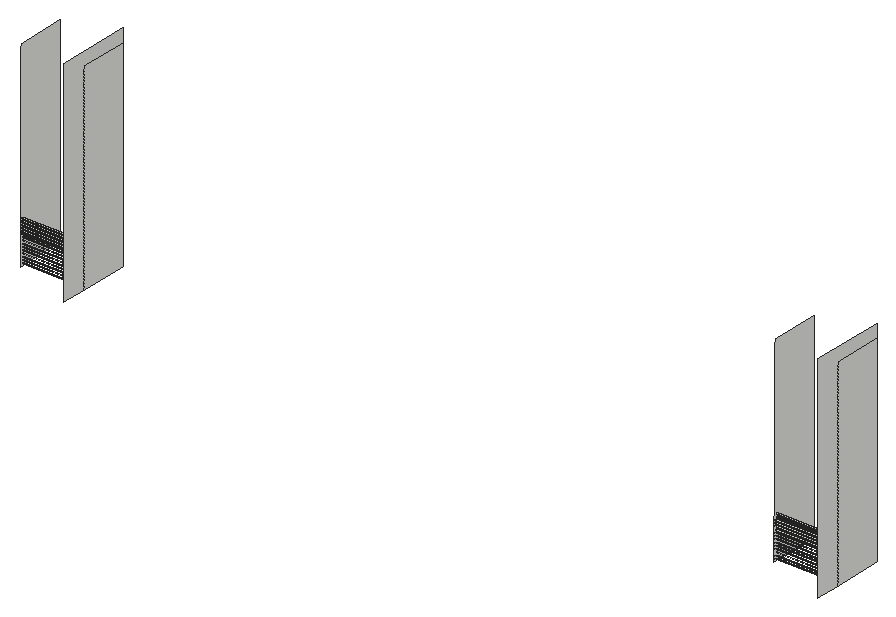
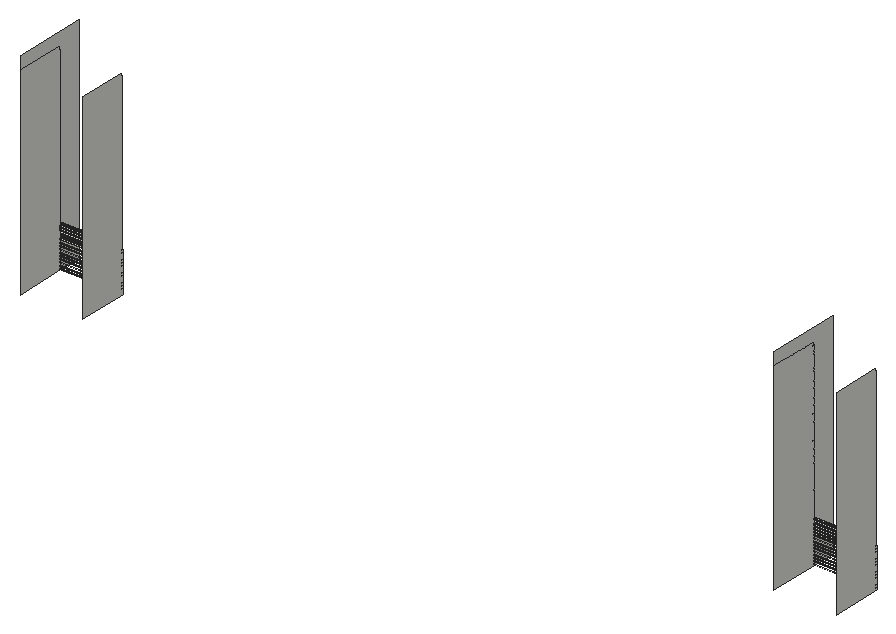
# SketchUp Ruby script. Lengths in inches.
U = 1.inch
M = Sketchup.active_model
def pt(a) = Geom::Point3d.new(a.map { |v| v * U })
def face(e, loops, mat)
  f = e.add_face(loops[0].map { |a| pt(a) })
  loops[1..].each { |l| e.add_face(l.map { |a| pt(a) }).erase! }
  f.material = f.back_material = mat if mat
  f
end
# faces: each face lists its corners as indices into pts; further lists are holes
def faces(e, pts, list, mat = nil) = list.each { |f| face(e, (f[0].is_a?(Array) ? f : [f]).map { |l| l.map { |i| pts[i] } }, mat) }
# xy, xz, yz: faces in a plane at the given z, y or x. An outline is a flat list of corners, or four numbers for a rectangle; further outlines are holes
def ring(l) = l.size == 4 ? [[l[0], l[1]], [l[2], l[1]], [l[2], l[3]], [l[0], l[3]]] : l.each_slice(2).to_a
def flat(e, list, mat, &to3) = list.each { |f| face(e, (f[0].is_a?(Array) ? f : [f]).map { |l| ring(l).map { |u, v| to3.(u, v) } }, mat) }
def xy(e, z, list, mat = nil) = flat(e, list, mat) { |x, y| [x, y, z] }
def xz(e, y, list, mat = nil) = flat(e, list, mat) { |x, z| [x, y, z] }
def yz(e, x, list, mat = nil) = flat(e, list, mat) { |y, z| [x, y, z] }
def lines(e, pts, list) = list.each { |a, b| e.add_line(pt(pts[a]), pt(pts[b])) }
# prism: a flat outline (further loops are holes) pulled along v
def prism(e, loops, v, mat = nil)
  f = face(e, loops, mat); d = Geom::Vector3d.new(v.map { |x| x * U })
  f.pushpull(f.normal.samedirection?(d) ? d.length : -d.length)
end
def box(e, o, s, mat = nil) = prism(e, [[o, [o[0] + s[0], o[1], o[2]], [o[0] + s[0], o[1] + s[1], o[2]], [o[0], o[1] + s[1], o[2]]]], [0, 0, s[2]], mat)
def at(x, y, z, deg = 0) = Geom::Transformation.translation(pt([x, y, z])) * Geom::Transformation.rotation(ORIGIN, Z_AXIS, deg.degrees)
def axes(o, x, y, z) = Geom::Transformation.new([*x, 0, *y, 0, *z, 0, *pt(o).to_a, 1])
def part(name) = M.definitions.add(name)
# library, detail: a bought-in or finely detailed component or shape, given as its bounding box
def library(name, o, s) = part(name).tap { |d| box(d.entities, o, s) }
def detail(e, o, s) = box(e.add_group.entities, o, s)
def put(e, d, t, mat = nil) = e.add_instance(d, t).tap { |i| i.material = mat if mat }
def group(e, t, mat = nil) = e.add_group.tap { |g| g.transformation = t; g.material = mat if mat }.entities
root = M.entities
xy(root,243.875,[[533.89,1125.04,620.51,1127.73],[1582.21,1125.04,1668.82,1127.73]])
xy(root,246.91,[[533.89,1125.04,620.51,1127.73],[1582.21,1125.04,1668.82,1127.73]])
xy(root,247.9375,[[533.89,1125.04,620.51,1127.73],[1582.21,1125.04,1668.82,1127.73]])
xy(root,250.97,[[533.89,1125.04,620.51,1127.73],[1582.21,1125.04,1668.82,1127.73]])
xy(root,252,[[533.89,1125.04,620.51,1127.73],[1582.21,1125.04,1668.82,1127.73]])
xy(root,255.03,[[533.89,1125.04,620.51,1127.73],[1582.21,1125.04,1668.82,1127.73]])
xy(root,256.0625,[[533.89,1125.04,620.51,1127.73],[1582.21,1125.04,1668.82,1127.73]])
xy(root,259.09,[[533.89,1125.04,620.51,1127.73],[1582.21,1125.04,1668.82,1127.73]])
xy(root,260.125,[[533.89,1125.42,620.51,1127.73],[1582.21,1125.42,1668.82,1127.73]])
xy(root,263.16,[[533.89,1125.42,620.51,1127.73],[1582.21,1125.42,1668.82,1127.73]])
xy(root,264.1875,[[533.89,1125.42,620.51,1127.73],[1582.21,1125.42,1668.82,1127.73]])
xz(root,1127.73,[[533.89,206.47,620.51,207.375],[1582.21,206.47,1668.82,207.375],[533.89,210.41,620.51,211.375],[1582.21,210.41,1668.82,211.375],[533.89,214.41,620.51,215.4375],
  [1582.21,214.41,1668.82,215.4375],[533.89,218.47,620.51,219.5],[1582.21,218.47,1668.82,219.5],[533.89,222.53,620.51,223.5625],[1582.21,222.53,1668.82,223.5625],
  [533.89,226.59,620.51,227.625],[1582.21,226.59,1668.82,227.625],[533.89,230.66,620.51,231.6875],[1582.21,230.66,1668.82,231.6875],[533.89,234.72,620.51,235.75],
  [1582.21,234.72,1668.82,235.75],[533.89,238.78,620.51,239.8125],[1582.21,238.78,1668.82,239.8125],[533.89,242.84,620.51,243.875]])
yz(root,533.89,[[1125.04,203.4375,1125.04,206.47,1127.73,206.47,1127.73,207.375,1125.04,207.375,1125.04,210.41,1127.73,210.41,1127.73,211.375,1125.04,211.375,1125.04,214.41,1127.73,214.41,1127.73,215.4375,1125.04,215.4375,1125.04,218.47,1127.73,218.47,1127.73,219.5,1125.04,219.5,1125.04,222.53,1127.73,222.53,1127.73,223.5625,1125.04,223.5625,1125.04,226.59,1127.73,226.59,1127.73,227.625,1125.04,227.625,1125.04,230.66,1127.73,230.66,1127.73,231.6875,1125.04,231.6875,1125.04,234.72,1127.73,234.72,1127.73,235.75,1125.04,235.75,1125.04,238.78,1127.73,238.78,1127.73,239.8125,1125.04,239.8125,1125.04,242.84,1127.73,242.84,1127.73,243.875,1125.04,243.875,1125.04,246.91,1127.73,246.91,1127.73,247.9375,1125.04,247.9375,1125.04,250.97,1127.73,250.97,1127.73,252,1125.04,252,1125.04,255.03,1127.73,255.03,1127.73,256.0625,1125.04,256.0625,1125.04,259.09,1127.73,259.09,1127.73,260.125,1125.42,260.125,1125.42,263.16,1127.73,263.16,1127.73,264.1875,1125.42,264.1875,1125.42,267.22,1127.73,267.22,1127.73,268.25,1125.42,268.25,1125.42,271.28,1127.73,271.28,1127.73,272.3125,1125.42,272.3125,1125.42,275.34,1127.73,275.34,1127.73,276.375,1125.42,276.375,1125.42,279.41,1127.73,279.41,1127.73,280.4375,1125.42,280.4375,1125.42,283.47,1127.73,283.47,1127.73,284.5,1125.42,284.5,1125.42,287.53,1127.73,287.53,1127.73,288.5625,1125.42,288.5625,1125.42,291.59,1127.73,291.59,1127.73,292.625,1125.42,292.625,1125.42,295.66,1127.73,295.66,1127.73,296.6875,1125.42,296.6875,1125.42,299.72,1127.73,299.72,1127.73,300.75,1125.42,300.75,1125.42,303.78,1127.73,303.78,1127.73,304.8125,1125.42,304.8125,1125.42,307.84,1127.73,307.84,1127.73,308.875,1125.42,308.875,1125.42,311.91,1127.73,311.91,1127.73,312.9375,1125.42,312.9375,1125.42,315.97,1127.73,315.97,1127.73,317,1125.42,317,1125.42,320.03,1127.73,320.03,1127.73,321.0625,1125.42,321.0625,1125.42,324.09,1127.73,324.09,1127.73,325.125,1125.42,325.125,1125.42,328.16,1127.73,328.16,1127.73,329.1875,1125.42,329.1875,1125.42,332.22,1127.73,332.22,1127.73,333.25,1125.42,333.25,1125.42,336.28,1127.73,336.28,1127.73,337.3125,1125.42,337.3125,1125.42,340.34,1127.73,340.34,1127.73,341.375,1125.42,341.375,1125.42,344.41,1127.73,344.41,1127.73,345.4375,1125.42,345.4375,1125.42,348.47,1127.73,348.47,1127.73,349.5,1125.42,349.5,1125.42,352.53,1127.73,352.53,1127.73,353.5625,1125.42,353.5625,1125.42,356.59,1127.73,356.59,1127.73,357.625,1125.42,357.625,1125.42,360.66,1127.73,360.66,1127.73,361.6875,1125.42,361.6875,1125.42,364.72,1127.73,364.72,1127.73,365.75,1125.42,365.75,1125.42,368.78,1127.73,368.78,1127.73,369.8125,1125.42,369.8125,1125.42,372.84,1127.73,372.84,1127.73,373.875,1125.42,373.875,1125.42,376.91,1127.73,376.91,1127.73,377.9375,1125.42,377.9375,1125.42,380.97,1127.73,380.97,1127.73,382,1125.42,382,1125.42,385.03,1127.73,385.03,1127.73,386.0625,1125.42,386.0625,1125.42,389.09,1127.73,389.09,1127.73,390.125,1125.42,390.125,1125.42,393.16,1127.73,393.16,1127.73,394.1875,1125.42,394.1875,1125.42,397.22,1127.73,397.22,1127.73,398.25,1125.42,398.25,1125.42,401.28,1127.73,401.28,1127.73,402.3125,1125.42,402.3125,1125.42,405.34,1127.73,405.34,1127.73,406.375,1125.42,406.375,1125.42,409.41,1127.73,409.41,1127.73,410.4375,1125.42,410.4375,1125.42,413.47,1127.73,413.47,1127.73,414.5,1125.42,414.5,1125.42,417.53,1127.73,417.53,1127.73,418.5625,1125.42,418.5625,1125.42,421.59,1127.73,421.59,1127.73,422.625,1125.42,422.625,1125.42,425.66,1127.73,425.66,1127.73,426.6875,1125.42,426.6875,1125.42,429.72,1127.73,429.72,1127.73,430.75,1125.42,430.75,1125.42,433.78,1127.73,433.78,1127.73,434.8125,1125.42,434.8125,1125.42,437.84,1127.73,437.84,1127.73,438.875,1125.42,438.875,1125.42,441.91,1127.73,441.91,1127.73,442.9375,1125.42,442.9375,1125.42,445.97,1127.73,445.97,1127.73,447,1125.42,447,1125.42,450.03,1127.73,450.03,1127.73,451.0625,1125.42,451.0625,1125.42,454.09,1127.73,454.09,1127.73,455.125,1125.42,455.125,1125.42,458.16,1127.73,458.16,1127.73,459.1875,1125.42,459.1875,1125.42,462.22,1127.73,462.22,1127.73,463.25,1125.42,463.25,1125.42,466.28,1127.73,466.28,1127.73,467.3125,1125.42,467.3125,1125.42,470.34,1127.73,470.34,1127.73,471.375,1125.42,471.375,1125.42,474.41,1127.73,474.41,1127.73,475.4375,1125.42,475.4375,1125.42,476.38,1127.73,476.38,1127.73,480,1194.07,480,1194.07,203.4375]])
yz(root,620.51,[[1092.87,203.4375,1092.87,500.5,1194.07,500.5,1194.07,482.53,1127.73,482.53,1127.73,478.47,1125.42,478.47,1125.42,475.4375,1127.73,475.4375,1127.73,474.41,1125.42,474.41,1125.42,471.375,1127.73,471.375,1127.73,470.34,1125.42,470.34,1125.42,467.3125,1127.73,467.3125,1127.73,466.28,1125.42,466.28,1125.42,463.25,1127.73,463.25,1127.73,462.22,1125.42,462.22,1125.42,459.1875,1127.73,459.1875,1127.73,458.16,1125.42,458.16,1125.42,455.125,1127.73,455.125,1127.73,454.09,1125.42,454.09,1125.42,451.0625,1127.73,451.0625,1127.73,450.03,1125.42,450.03,1125.42,447,1127.73,447,1127.73,445.97,1125.42,445.97,1125.42,442.9375,1127.73,442.9375,1127.73,441.91,1125.42,441.91,1125.42,438.875,1127.73,438.875,1127.73,437.84,1125.42,437.84,1125.42,434.8125,1127.73,434.8125,1127.73,433.78,1125.42,433.78,1125.42,430.75,1127.73,430.75,1127.73,429.72,1125.42,429.72,1125.42,426.6875,1127.73,426.6875,1127.73,425.66,1125.42,425.66,1125.42,422.625,1127.73,422.625,1127.73,421.59,1125.42,421.59,1125.42,418.5625,1127.73,418.5625,1127.73,417.53,1125.42,417.53,1125.42,414.5,1127.73,414.5,1127.73,413.47,1125.42,413.47,1125.42,410.4375,1127.73,410.4375,1127.73,409.41,1125.42,409.41,1125.42,406.375,1127.73,406.375,1127.73,405.34,1125.42,405.34,1125.42,402.3125,1127.73,402.3125,1127.73,401.28,1125.42,401.28,1125.42,398.25,1127.73,398.25,1127.73,397.22,1125.42,397.22,1125.42,394.1875,1127.73,394.1875,1127.73,393.16,1125.42,393.16,1125.42,390.125,1127.73,390.125,1127.73,389.09,1125.42,389.09,1125.42,386.0625,1127.73,386.0625,1127.73,385.03,1125.42,385.03,1125.42,382,1127.73,382,1127.73,380.97,1125.42,380.97,1125.42,377.9375,1127.73,377.9375,1127.73,376.91,1125.42,376.91,1125.42,373.875,1127.73,373.875,1127.73,372.84,1125.42,372.84,1125.42,369.8125,1127.73,369.8125,1127.73,368.78,1125.42,368.78,1125.42,365.75,1127.73,365.75,1127.73,364.72,1125.42,364.72,1125.42,361.6875,1127.73,361.6875,1127.73,360.66,1125.42,360.66,1125.42,357.625,1127.73,357.625,1127.73,356.59,1125.42,356.59,1125.42,353.5625,1127.73,353.5625,1127.73,352.53,1125.42,352.53,1125.42,349.5,1127.73,349.5,1127.73,348.47,1125.42,348.47,1125.42,345.4375,1127.73,345.4375,1127.73,344.41,1125.42,344.41,1125.42,341.375,1127.73,341.375,1127.73,340.34,1125.42,340.34,1125.42,337.3125,1127.73,337.3125,1127.73,336.28,1125.42,336.28,1125.42,333.25,1127.73,333.25,1127.73,332.22,1125.42,332.22,1125.42,329.1875,1127.73,329.1875,1127.73,328.16,1125.42,328.16,1125.42,325.125,1127.73,325.125,1127.73,324.09,1125.42,324.09,1125.42,321.0625,1127.73,321.0625,1127.73,320.03,1125.42,320.03,1125.42,317,1127.73,317,1127.73,315.97,1125.42,315.97,1125.42,312.9375,1127.73,312.9375,1127.73,311.91,1125.42,311.91,1125.42,308.875,1127.73,308.875,1127.73,307.84,1125.42,307.84,1125.42,304.8125,1127.73,304.8125,1127.73,303.78,1125.42,303.78,1125.42,300.75,1127.73,300.75,1127.73,299.72,1125.42,299.72,1125.42,296.6875,1127.73,296.6875,1127.73,295.66,1125.42,295.66,1125.42,292.625,1127.73,292.625,1127.73,291.59,1125.42,291.59,1125.42,288.5625,1127.73,288.5625,1127.73,287.53,1125.42,287.53,1125.42,284.5,1127.73,284.5,1127.73,283.47,1125.42,283.47,1125.42,280.4375,1127.73,280.4375,1127.73,279.41,1125.42,279.41,1125.42,276.375,1127.73,276.375,1127.73,275.34,1125.42,275.34,1125.42,272.3125,1127.73,272.3125,1127.73,271.28,1125.42,271.28,1125.42,268.25,1127.73,268.25,1127.73,267.22,1125.42,267.22,1125.42,264.1875,1127.73,264.1875,1127.73,263.16,1125.42,263.16,1125.42,260.125,1127.73,260.125,1127.73,259.09,1125.04,259.09,1125.04,256.0625,1127.73,256.0625,1127.73,255.03,1125.04,255.03,1125.04,252,1127.73,252,1127.73,250.97,1125.04,250.97,1125.04,247.9375,1127.73,247.9375,1127.73,246.91,1125.04,246.91,1125.04,243.875,1127.73,243.875,1127.73,242.84,1125.04,242.84,1125.04,239.8125,1127.73,239.8125,1127.73,238.78,1125.04,238.78,1125.04,235.75,1127.73,235.75,1127.73,234.72,1125.04,234.72,1125.04,231.6875,1127.73,231.6875,1127.73,230.66,1125.04,230.66,1125.04,227.625,1127.73,227.625,1127.73,226.59,1125.04,226.59,1125.04,223.5625,1127.73,223.5625,1127.73,222.53,1125.04,222.53,1125.04,219.5,1127.73,219.5,1127.73,218.47,1125.04,218.47,1125.04,215.4375,1127.73,215.4375,1127.73,214.41,1125.04,214.41,1125.04,211.375,1127.73,211.375,1127.73,210.41,1125.04,210.41,1125.04,207.375,1127.73,207.375,1127.73,206.47,1125.04,206.47,1125.04,203.4375],[1125.04,203.4375,1125.04,206.47,1127.73,206.47,1127.73,207.375,1125.04,207.375,1125.04,210.41,1127.73,210.41,1127.73,211.375,1125.04,211.375,1125.04,214.41,1127.73,214.41,1127.73,215.4375,1125.04,215.4375,1125.04,218.47,1127.73,218.47,1127.73,219.5,1125.04,219.5,1125.04,222.53,1127.73,222.53,1127.73,223.5625,1125.04,223.5625,1125.04,226.59,1127.73,226.59,1127.73,227.625,1125.04,227.625,1125.04,230.66,1127.73,230.66,1127.73,231.6875,1125.04,231.6875,1125.04,234.72,1127.73,234.72,1127.73,235.75,1125.04,235.75,1125.04,238.78,1127.73,238.78,1127.73,239.8125,1125.04,239.8125,1125.04,242.84,1127.73,242.84,1127.73,243.875,1125.04,243.875,1125.04,246.91,1127.73,246.91,1127.73,247.9375,1125.04,247.9375,1125.04,250.97,1127.73,250.97,1127.73,252,1125.04,252,1125.04,255.03,1127.73,255.03,1127.73,256.0625,1125.04,256.0625,1125.04,259.09,1127.73,259.09,1127.73,260.125,1125.42,260.125,1125.42,263.16,1127.73,263.16,1127.73,264.1875,1125.42,264.1875,1125.42,267.22,1127.73,267.22,1127.73,268.25,1125.42,268.25,1125.42,271.28,1127.73,271.28,1127.73,272.3125,1125.42,272.3125,1125.42,275.34,1127.73,275.34,1127.73,276.375,1125.42,276.375,1125.42,279.41,1127.73,279.41,1127.73,280.4375,1125.42,280.4375,1125.42,283.47,1127.73,283.47,1127.73,284.5,1125.42,284.5,1125.42,287.53,1127.73,287.53,1127.73,288.5625,1125.42,288.5625,1125.42,291.59,1127.73,291.59,1127.73,292.625,1125.42,292.625,1125.42,295.66,1127.73,295.66,1127.73,296.6875,1125.42,296.6875,1125.42,299.72,1127.73,299.72,1127.73,300.75,1125.42,300.75,1125.42,303.78,1127.73,303.78,1127.73,304.8125,1125.42,304.8125,1125.42,307.84,1127.73,307.84,1127.73,308.875,1125.42,308.875,1125.42,311.91,1127.73,311.91,1127.73,312.9375,1125.42,312.9375,1125.42,315.97,1127.73,315.97,1127.73,317,1125.42,317,1125.42,320.03,1127.73,320.03,1127.73,321.0625,1125.42,321.0625,1125.42,324.09,1127.73,324.09,1127.73,325.125,1125.42,325.125,1125.42,328.16,1127.73,328.16,1127.73,329.1875,1125.42,329.1875,1125.42,332.22,1127.73,332.22,1127.73,333.25,1125.42,333.25,1125.42,336.28,1127.73,336.28,1127.73,337.3125,1125.42,337.3125,1125.42,340.34,1127.73,340.34,1127.73,341.375,1125.42,341.375,1125.42,344.41,1127.73,344.41,1127.73,345.4375,1125.42,345.4375,1125.42,348.47,1127.73,348.47,1127.73,349.5,1125.42,349.5,1125.42,352.53,1127.73,352.53,1127.73,353.5625,1125.42,353.5625,1125.42,356.59,1127.73,356.59,1127.73,357.625,1125.42,357.625,1125.42,360.66,1127.73,360.66,1127.73,361.6875,1125.42,361.6875,1125.42,364.72,1127.73,364.72,1127.73,365.75,1125.42,365.75,1125.42,368.78,1127.73,368.78,1127.73,369.8125,1125.42,369.8125,1125.42,372.84,1127.73,372.84,1127.73,373.875,1125.42,373.875,1125.42,376.91,1127.73,376.91,1127.73,377.9375,1125.42,377.9375,1125.42,380.97,1127.73,380.97,1127.73,382,1125.42,382,1125.42,385.03,1127.73,385.03,1127.73,386.0625,1125.42,386.0625,1125.42,389.09,1127.73,389.09,1127.73,390.125,1125.42,390.125,1125.42,393.16,1127.73,393.16,1127.73,394.1875,1125.42,394.1875,1125.42,397.22,1127.73,397.22,1127.73,398.25,1125.42,398.25,1125.42,401.28,1127.73,401.28,1127.73,402.3125,1125.42,402.3125,1125.42,405.34,1127.73,405.34,1127.73,406.375,1125.42,406.375,1125.42,409.41,1127.73,409.41,1127.73,410.4375,1125.42,410.4375,1125.42,413.47,1127.73,413.47,1127.73,414.5,1125.42,414.5,1125.42,417.53,1127.73,417.53,1127.73,418.5625,1125.42,418.5625,1125.42,421.59,1127.73,421.59,1127.73,422.625,1125.42,422.625,1125.42,425.66,1127.73,425.66,1127.73,426.6875,1125.42,426.6875,1125.42,429.72,1127.73,429.72,1127.73,430.75,1125.42,430.75,1125.42,433.78,1127.73,433.78,1127.73,434.8125,1125.42,434.8125,1125.42,437.84,1127.73,437.84,1127.73,438.875,1125.42,438.875,1125.42,441.91,1127.73,441.91,1127.73,442.9375,1125.42,442.9375,1125.42,445.97,1127.73,445.97,1127.73,447,1125.42,447,1125.42,450.03,1127.73,450.03,1127.73,451.0625,1125.42,451.0625,1125.42,454.09,1127.73,454.09,1127.73,455.125,1125.42,455.125,1125.42,458.16,1127.73,458.16,1127.73,459.1875,1125.42,459.1875,1125.42,462.22,1127.73,462.22,1127.73,463.25,1125.42,463.25,1125.42,466.28,1127.73,466.28,1127.73,467.3125,1125.42,467.3125,1125.42,470.34,1127.73,470.34,1127.73,471.375,1125.42,471.375,1125.42,474.41,1127.73,474.41,1127.73,475.4375,1125.42,475.4375,1125.42,478.47,1127.73,478.47,1127.73,482.53,1194.07,482.53,1194.07,203.4375]])
yz(root,1582.21,[[1125.04,203.4375,1125.04,206.47,1127.73,206.47,1127.73,207.375,1125.04,207.375,1125.04,210.41,1127.73,210.41,1127.73,211.375,1125.04,211.375,1125.04,214.41,1127.73,214.41,1127.73,215.4375,1125.04,215.4375,1125.04,218.47,1127.73,218.47,1127.73,219.5,1125.04,219.5,1125.04,222.53,1127.73,222.53,1127.73,223.5625,1125.04,223.5625,1125.04,226.59,1127.73,226.59,1127.73,227.625,1125.04,227.625,1125.04,230.66,1127.73,230.66,1127.73,231.6875,1125.04,231.6875,1125.04,234.72,1127.73,234.72,1127.73,235.75,1125.04,235.75,1125.04,238.78,1127.73,238.78,1127.73,239.8125,1125.04,239.8125,1125.04,242.84,1127.73,242.84,1127.73,243.875,1125.04,243.875,1125.04,246.91,1127.73,246.91,1127.73,247.9375,1125.04,247.9375,1125.04,250.97,1127.73,250.97,1127.73,252,1125.04,252,1125.04,255.03,1127.73,255.03,1127.73,256.0625,1125.04,256.0625,1125.04,259.09,1127.73,259.09,1127.73,260.125,1125.42,260.125,1125.42,263.16,1127.73,263.16,1127.73,264.1875,1125.42,264.1875,1125.42,267.22,1127.73,267.22,1127.73,268.25,1125.42,268.25,1125.42,271.28,1127.73,271.28,1127.73,272.3125,1125.42,272.3125,1125.42,275.34,1127.73,275.34,1127.73,276.375,1125.42,276.375,1125.42,279.41,1127.73,279.41,1127.73,280.4375,1125.42,280.4375,1125.42,283.47,1127.73,283.47,1127.73,284.5,1125.42,284.5,1125.42,287.53,1127.73,287.53,1127.73,288.5625,1125.42,288.5625,1125.42,291.59,1127.73,291.59,1127.73,292.625,1125.42,292.625,1125.42,295.66,1127.73,295.66,1127.73,296.6875,1125.42,296.6875,1125.42,299.72,1127.73,299.72,1127.73,300.75,1125.42,300.75,1125.42,303.78,1127.73,303.78,1127.73,304.8125,1125.42,304.8125,1125.42,307.84,1127.73,307.84,1127.73,308.875,1125.42,308.875,1125.42,311.91,1127.73,311.91,1127.73,312.9375,1125.42,312.9375,1125.42,315.97,1127.73,315.97,1127.73,317,1125.42,317,1125.42,320.03,1127.73,320.03,1127.73,321.0625,1125.42,321.0625,1125.42,324.09,1127.73,324.09,1127.73,325.125,1125.42,325.125,1125.42,328.16,1127.73,328.16,1127.73,329.1875,1125.42,329.1875,1125.42,332.22,1127.73,332.22,1127.73,333.25,1125.42,333.25,1125.42,336.28,1127.73,336.28,1127.73,337.3125,1125.42,337.3125,1125.42,340.34,1127.73,340.34,1127.73,341.375,1125.42,341.375,1125.42,344.41,1127.73,344.41,1127.73,345.4375,1125.42,345.4375,1125.42,348.47,1127.73,348.47,1127.73,349.5,1125.42,349.5,1125.42,352.53,1127.73,352.53,1127.73,353.5625,1125.42,353.5625,1125.42,356.59,1127.73,356.59,1127.73,357.625,1125.42,357.625,1125.42,360.66,1127.73,360.66,1127.73,361.6875,1125.42,361.6875,1125.42,364.72,1127.73,364.72,1127.73,365.75,1125.42,365.75,1125.42,368.78,1127.73,368.78,1127.73,369.8125,1125.42,369.8125,1125.42,372.84,1127.73,372.84,1127.73,373.875,1125.42,373.875,1125.42,376.91,1127.73,376.91,1127.73,377.9375,1125.42,377.9375,1125.42,380.97,1127.73,380.97,1127.73,382,1125.42,382,1125.42,385.03,1127.73,385.03,1127.73,386.0625,1125.42,386.0625,1125.42,389.09,1127.73,389.09,1127.73,390.125,1125.42,390.125,1125.42,393.16,1127.73,393.16,1127.73,394.1875,1125.42,394.1875,1125.42,397.22,1127.73,397.22,1127.73,398.25,1125.42,398.25,1125.42,401.28,1127.73,401.28,1127.73,402.3125,1125.42,402.3125,1125.42,405.34,1127.73,405.34,1127.73,406.375,1125.42,406.375,1125.42,409.41,1127.73,409.41,1127.73,410.4375,1125.42,410.4375,1125.42,413.47,1127.73,413.47,1127.73,414.5,1125.42,414.5,1125.42,417.53,1127.73,417.53,1127.73,418.5625,1125.42,418.5625,1125.42,421.59,1127.73,421.59,1127.73,422.625,1125.42,422.625,1125.42,425.66,1127.73,425.66,1127.73,426.6875,1125.42,426.6875,1125.42,429.72,1127.73,429.72,1127.73,430.75,1125.42,430.75,1125.42,433.78,1127.73,433.78,1127.73,434.8125,1125.42,434.8125,1125.42,437.84,1127.73,437.84,1127.73,438.875,1125.42,438.875,1125.42,441.91,1127.73,441.91,1127.73,442.9375,1125.42,442.9375,1125.42,445.97,1127.73,445.97,1127.73,447,1125.42,447,1125.42,450.03,1127.73,450.03,1127.73,451.0625,1125.42,451.0625,1125.42,454.09,1127.73,454.09,1127.73,455.125,1125.42,455.125,1125.42,458.16,1127.73,458.16,1127.73,459.1875,1125.42,459.1875,1125.42,462.22,1127.73,462.22,1127.73,463.25,1125.42,463.25,1125.42,466.28,1127.73,466.28,1127.73,467.3125,1125.42,467.3125,1125.42,470.34,1127.73,470.34,1127.73,471.375,1125.42,471.375,1125.42,474.41,1127.73,474.41,1127.73,475.4375,1125.42,475.4375,1125.42,476.38,1127.73,476.38,1127.73,480,1194.07,480,1194.07,203.4375]])
yz(root,1668.82,[[1092.87,203.4375,1092.87,500.5,1194.07,500.5,1194.07,482.53,1127.73,482.53,1127.73,478.47,1125.42,478.47,1125.42,475.4375,1127.73,475.4375,1127.73,474.41,1125.42,474.41,1125.42,471.375,1127.73,471.375,1127.73,470.34,1125.42,470.34,1125.42,467.3125,1127.73,467.3125,1127.73,466.28,1125.42,466.28,1125.42,463.25,1127.73,463.25,1127.73,462.22,1125.42,462.22,1125.42,459.1875,1127.73,459.1875,1127.73,458.16,1125.42,458.16,1125.42,455.125,1127.73,455.125,1127.73,454.09,1125.42,454.09,1125.42,451.0625,1127.73,451.0625,1127.73,450.03,1125.42,450.03,1125.42,447,1127.73,447,1127.73,445.97,1125.42,445.97,1125.42,442.9375,1127.73,442.9375,1127.73,441.91,1125.42,441.91,1125.42,438.875,1127.73,438.875,1127.73,437.84,1125.42,437.84,1125.42,434.8125,1127.73,434.8125,1127.73,433.78,1125.42,433.78,1125.42,430.75,1127.73,430.75,1127.73,429.72,1125.42,429.72,1125.42,426.6875,1127.73,426.6875,1127.73,425.66,1125.42,425.66,1125.42,422.625,1127.73,422.625,1127.73,421.59,1125.42,421.59,1125.42,418.5625,1127.73,418.5625,1127.73,417.53,1125.42,417.53,1125.42,414.5,1127.73,414.5,1127.73,413.47,1125.42,413.47,1125.42,410.4375,1127.73,410.4375,1127.73,409.41,1125.42,409.41,1125.42,406.375,1127.73,406.375,1127.73,405.34,1125.42,405.34,1125.42,402.3125,1127.73,402.3125,1127.73,401.28,1125.42,401.28,1125.42,398.25,1127.73,398.25,1127.73,397.22,1125.42,397.22,1125.42,394.1875,1127.73,394.1875,1127.73,393.16,1125.42,393.16,1125.42,390.125,1127.73,390.125,1127.73,389.09,1125.42,389.09,1125.42,386.0625,1127.73,386.0625,1127.73,385.03,1125.42,385.03,1125.42,382,1127.73,382,1127.73,380.97,1125.42,380.97,1125.42,377.9375,1127.73,377.9375,1127.73,376.91,1125.42,376.91,1125.42,373.875,1127.73,373.875,1127.73,372.84,1125.42,372.84,1125.42,369.8125,1127.73,369.8125,1127.73,368.78,1125.42,368.78,1125.42,365.75,1127.73,365.75,1127.73,364.72,1125.42,364.72,1125.42,361.6875,1127.73,361.6875,1127.73,360.66,1125.42,360.66,1125.42,357.625,1127.73,357.625,1127.73,356.59,1125.42,356.59,1125.42,353.5625,1127.73,353.5625,1127.73,352.53,1125.42,352.53,1125.42,349.5,1127.73,349.5,1127.73,348.47,1125.42,348.47,1125.42,345.4375,1127.73,345.4375,1127.73,344.41,1125.42,344.41,1125.42,341.375,1127.73,341.375,1127.73,340.34,1125.42,340.34,1125.42,337.3125,1127.73,337.3125,1127.73,336.28,1125.42,336.28,1125.42,333.25,1127.73,333.25,1127.73,332.22,1125.42,332.22,1125.42,329.1875,1127.73,329.1875,1127.73,328.16,1125.42,328.16,1125.42,325.125,1127.73,325.125,1127.73,324.09,1125.42,324.09,1125.42,321.0625,1127.73,321.0625,1127.73,320.03,1125.42,320.03,1125.42,317,1127.73,317,1127.73,315.97,1125.42,315.97,1125.42,312.9375,1127.73,312.9375,1127.73,311.91,1125.42,311.91,1125.42,308.875,1127.73,308.875,1127.73,307.84,1125.42,307.84,1125.42,304.8125,1127.73,304.8125,1127.73,303.78,1125.42,303.78,1125.42,300.75,1127.73,300.75,1127.73,299.72,1125.42,299.72,1125.42,296.6875,1127.73,296.6875,1127.73,295.66,1125.42,295.66,1125.42,292.625,1127.73,292.625,1127.73,291.59,1125.42,291.59,1125.42,288.5625,1127.73,288.5625,1127.73,287.53,1125.42,287.53,1125.42,284.5,1127.73,284.5,1127.73,283.47,1125.42,283.47,1125.42,280.4375,1127.73,280.4375,1127.73,279.41,1125.42,279.41,1125.42,276.375,1127.73,276.375,1127.73,275.34,1125.42,275.34,1125.42,272.3125,1127.73,272.3125,1127.73,271.28,1125.42,271.28,1125.42,268.25,1127.73,268.25,1127.73,267.22,1125.42,267.22,1125.42,264.1875,1127.73,264.1875,1127.73,263.16,1125.42,263.16,1125.42,260.125,1127.73,260.125,1127.73,259.09,1125.04,259.09,1125.04,256.0625,1127.73,256.0625,1127.73,255.03,1125.04,255.03,1125.04,252,1127.73,252,1127.73,250.97,1125.04,250.97,1125.04,247.9375,1127.73,247.9375,1127.73,246.91,1125.04,246.91,1125.04,243.875,1127.73,243.875,1127.73,242.84,1125.04,242.84,1125.04,239.8125,1127.73,239.8125,1127.73,238.78,1125.04,238.78,1125.04,235.75,1127.73,235.75,1127.73,234.72,1125.04,234.72,1125.04,231.6875,1127.73,231.6875,1127.73,230.66,1125.04,230.66,1125.04,227.625,1127.73,227.625,1127.73,226.59,1125.04,226.59,1125.04,223.5625,1127.73,223.5625,1127.73,222.53,1125.04,222.53,1125.04,219.5,1127.73,219.5,1127.73,218.47,1125.04,218.47,1125.04,215.4375,1127.73,215.4375,1127.73,214.41,1125.04,214.41,1125.04,211.375,1127.73,211.375,1127.73,210.41,1125.04,210.41,1125.04,207.375,1127.73,207.375,1127.73,206.47,1125.04,206.47,1125.04,203.4375],[1125.04,203.4375,1125.04,206.47,1127.73,206.47,1127.73,207.375,1125.04,207.375,1125.04,210.41,1127.73,210.41,1127.73,211.375,1125.04,211.375,1125.04,214.41,1127.73,214.41,1127.73,215.4375,1125.04,215.4375,1125.04,218.47,1127.73,218.47,1127.73,219.5,1125.04,219.5,1125.04,222.53,1127.73,222.53,1127.73,223.5625,1125.04,223.5625,1125.04,226.59,1127.73,226.59,1127.73,227.625,1125.04,227.625,1125.04,230.66,1127.73,230.66,1127.73,231.6875,1125.04,231.6875,1125.04,234.72,1127.73,234.72,1127.73,235.75,1125.04,235.75,1125.04,238.78,1127.73,238.78,1127.73,239.8125,1125.04,239.8125,1125.04,242.84,1127.73,242.84,1127.73,243.875,1125.04,243.875,1125.04,246.91,1127.73,246.91,1127.73,247.9375,1125.04,247.9375,1125.04,250.97,1127.73,250.97,1127.73,252,1125.04,252,1125.04,255.03,1127.73,255.03,1127.73,256.0625,1125.04,256.0625,1125.04,259.09,1127.73,259.09,1127.73,260.125,1125.42,260.125,1125.42,263.16,1127.73,263.16,1127.73,264.1875,1125.42,264.1875,1125.42,267.22,1127.73,267.22,1127.73,268.25,1125.42,268.25,1125.42,271.28,1127.73,271.28,1127.73,272.3125,1125.42,272.3125,1125.42,275.34,1127.73,275.34,1127.73,276.375,1125.42,276.375,1125.42,279.41,1127.73,279.41,1127.73,280.4375,1125.42,280.4375,1125.42,283.47,1127.73,283.47,1127.73,284.5,1125.42,284.5,1125.42,287.53,1127.73,287.53,1127.73,288.5625,1125.42,288.5625,1125.42,291.59,1127.73,291.59,1127.73,292.625,1125.42,292.625,1125.42,295.66,1127.73,295.66,1127.73,296.6875,1125.42,296.6875,1125.42,299.72,1127.73,299.72,1127.73,300.75,1125.42,300.75,1125.42,303.78,1127.73,303.78,1127.73,304.8125,1125.42,304.8125,1125.42,307.84,1127.73,307.84,1127.73,308.875,1125.42,308.875,1125.42,311.91,1127.73,311.91,1127.73,312.9375,1125.42,312.9375,1125.42,315.97,1127.73,315.97,1127.73,317,1125.42,317,1125.42,320.03,1127.73,320.03,1127.73,321.0625,1125.42,321.0625,1125.42,324.09,1127.73,324.09,1127.73,325.125,1125.42,325.125,1125.42,328.16,1127.73,328.16,1127.73,329.1875,1125.42,329.1875,1125.42,332.22,1127.73,332.22,1127.73,333.25,1125.42,333.25,1125.42,336.28,1127.73,336.28,1127.73,337.3125,1125.42,337.3125,1125.42,340.34,1127.73,340.34,1127.73,341.375,1125.42,341.375,1125.42,344.41,1127.73,344.41,1127.73,345.4375,1125.42,345.4375,1125.42,348.47,1127.73,348.47,1127.73,349.5,1125.42,349.5,1125.42,352.53,1127.73,352.53,1127.73,353.5625,1125.42,353.5625,1125.42,356.59,1127.73,356.59,1127.73,357.625,1125.42,357.625,1125.42,360.66,1127.73,360.66,1127.73,361.6875,1125.42,361.6875,1125.42,364.72,1127.73,364.72,1127.73,365.75,1125.42,365.75,1125.42,368.78,1127.73,368.78,1127.73,369.8125,1125.42,369.8125,1125.42,372.84,1127.73,372.84,1127.73,373.875,1125.42,373.875,1125.42,376.91,1127.73,376.91,1127.73,377.9375,1125.42,377.9375,1125.42,380.97,1127.73,380.97,1127.73,382,1125.42,382,1125.42,385.03,1127.73,385.03,1127.73,386.0625,1125.42,386.0625,1125.42,389.09,1127.73,389.09,1127.73,390.125,1125.42,390.125,1125.42,393.16,1127.73,393.16,1127.73,394.1875,1125.42,394.1875,1125.42,397.22,1127.73,397.22,1127.73,398.25,1125.42,398.25,1125.42,401.28,1127.73,401.28,1127.73,402.3125,1125.42,402.3125,1125.42,405.34,1127.73,405.34,1127.73,406.375,1125.42,406.375,1125.42,409.41,1127.73,409.41,1127.73,410.4375,1125.42,410.4375,1125.42,413.47,1127.73,413.47,1127.73,414.5,1125.42,414.5,1125.42,417.53,1127.73,417.53,1127.73,418.5625,1125.42,418.5625,1125.42,421.59,1127.73,421.59,1127.73,422.625,1125.42,422.625,1125.42,425.66,1127.73,425.66,1127.73,426.6875,1125.42,426.6875,1125.42,429.72,1127.73,429.72,1127.73,430.75,1125.42,430.75,1125.42,433.78,1127.73,433.78,1127.73,434.8125,1125.42,434.8125,1125.42,437.84,1127.73,437.84,1127.73,438.875,1125.42,438.875,1125.42,441.91,1127.73,441.91,1127.73,442.9375,1125.42,442.9375,1125.42,445.97,1127.73,445.97,1127.73,447,1125.42,447,1125.42,450.03,1127.73,450.03,1127.73,451.0625,1125.42,451.0625,1125.42,454.09,1127.73,454.09,1127.73,455.125,1125.42,455.125,1125.42,458.16,1127.73,458.16,1127.73,459.1875,1125.42,459.1875,1125.42,462.22,1127.73,462.22,1127.73,463.25,1125.42,463.25,1125.42,466.28,1127.73,466.28,1127.73,467.3125,1125.42,467.3125,1125.42,470.34,1127.73,470.34,1127.73,471.375,1125.42,471.375,1125.42,474.41,1127.73,474.41,1127.73,475.4375,1125.42,475.4375,1125.42,478.47,1127.73,478.47,1127.73,482.53,1194.07,482.53,1194.07,203.4375]])
